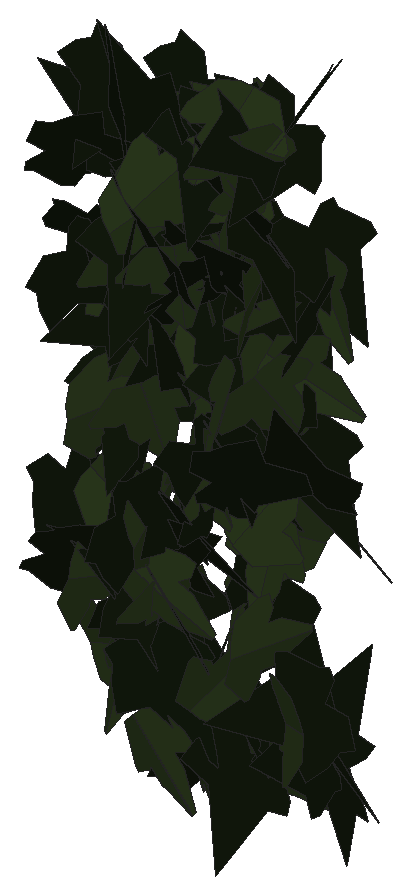
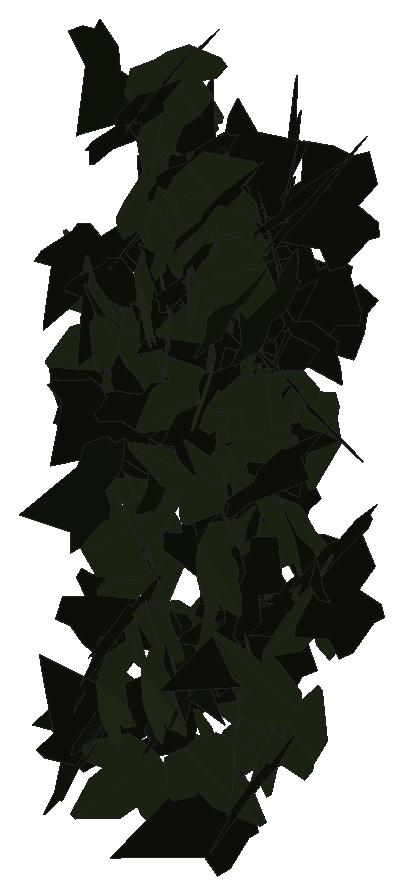
# SketchUp Ruby script. Lengths in inches.
U = 1.inch
M = Sketchup.active_model
def pt(a) = Geom::Point3d.new(a.map { |v| v * U })
def face(e, loops, mat)
  f = e.add_face(loops[0].map { |a| pt(a) })
  loops[1..].each { |l| e.add_face(l.map { |a| pt(a) }).erase! }
  f.material = f.back_material = mat if mat
  f
end
# faces: each face lists its corners as indices into pts; further lists are holes
def faces(e, pts, list, mat = nil) = list.each { |f| face(e, (f[0].is_a?(Array) ? f : [f]).map { |l| l.map { |i| pts[i] } }, mat) }
# xy, xz, yz: faces in a plane at the given z, y or x. An outline is a flat list of corners, or four numbers for a rectangle; further outlines are holes
def ring(l) = l.size == 4 ? [[l[0], l[1]], [l[2], l[1]], [l[2], l[3]], [l[0], l[3]]] : l.each_slice(2).to_a
def flat(e, list, mat, &to3) = list.each { |f| face(e, (f[0].is_a?(Array) ? f : [f]).map { |l| ring(l).map { |u, v| to3.(u, v) } }, mat) }
def xy(e, z, list, mat = nil) = flat(e, list, mat) { |x, y| [x, y, z] }
def xz(e, y, list, mat = nil) = flat(e, list, mat) { |x, z| [x, y, z] }
def yz(e, x, list, mat = nil) = flat(e, list, mat) { |y, z| [x, y, z] }
def lines(e, pts, list) = list.each { |a, b| e.add_line(pt(pts[a]), pt(pts[b])) }
# prism: a flat outline (further loops are holes) pulled along v
def prism(e, loops, v, mat = nil)
  f = face(e, loops, mat); d = Geom::Vector3d.new(v.map { |x| x * U })
  f.pushpull(f.normal.samedirection?(d) ? d.length : -d.length)
end
def box(e, o, s, mat = nil) = prism(e, [[o, [o[0] + s[0], o[1], o[2]], [o[0] + s[0], o[1] + s[1], o[2]], [o[0], o[1] + s[1], o[2]]]], [0, 0, s[2]], mat)
def at(x, y, z, deg = 0) = Geom::Transformation.translation(pt([x, y, z])) * Geom::Transformation.rotation(ORIGIN, Z_AXIS, deg.degrees)
def axes(o, x, y, z) = Geom::Transformation.new([*x, 0, *y, 0, *z, 0, *pt(o).to_a, 1])
def part(name) = M.definitions.add(name)
# library, detail: a bought-in or finely detailed component or shape, given as its bounding box
def library(name, o, s) = part(name).tap { |d| box(d.entities, o, s) }
def detail(e, o, s) = box(e.add_group.entities, o, s)
def put(e, d, t, mat = nil) = e.add_instance(d, t).tap { |i| i.material = mat if mat }
def group(e, t, mat = nil) = e.add_group.tap { |g| g.transformation = t; g.material = mat if mat }.entities
root = M.entities
M.materials.add("efeu1").color = [18, 25, 13]
M.materials.add("efeu2").color = [43, 57, 29]
c1 = part("ivyleaf_9")
p = [[1.54,2.16,1.25],[1.36,2.04,1.19],[-0.21,0.99,0.68],[-0.71,1.11,0.82],[-0.85,0.86,0.67],[-0.8,0.17,0.21],
  [-0.9,-0.01,0.1],[-0.67,-0.16,-0.02],[-0.08,-0.08,-0.05],[-0.03,-0.6,-0.4],[0.65,-0.88,-0.66],[0.83,-0.6,-0.49],
  [1.29,-0.42,-0.43],[1.8125,-0.07,-0.26],[1.21,0.44,0.15]]
faces(c1.entities,p,[[0,1,2,3,4,5,6,7,8,9,10,11,12,13,14]],"efeu1")
c2 = part("ivyleaf_10")
p = [[0,0.5,-0.03],[-0.0625,2.02,-0.43],[-0.19,2.01,-0.46],[-0.54,1.05,-0.29],[-0.52,0.625,-0.18],[-0.83,0.76,-0.28],
  [-1.16,0.64,-0.33],[-1.15,0.33,-0.24],[-0.77,-0.39,0.02],[-0.3,-0.51,0.16],[0.04,-0.48,0.23],[-0.02,2.01,-0.4375],
  [-0.06,2.01,-0.43],[0.04,-0.49,0.23],[0.67,-0.49,0.14],[1.38,0.36,-0.2],[1.375,0.51,-0.24],[0.81,0.65,-0.19],
  [0.62,0.59,-0.15],[0.6,1.09,-0.28],[0.5,1.23,-0.31]]
faces(c2.entities,p,[[0,1,2,3,4,5,6,7,8,9,10],[11,12,0,13,14,15,16,17,18,19,20]],"efeu2")
put(root,c1,axes([32.22,223.73,222.4],[-0.13186,-0.40837,0.25661],[-0.00992,-0.26368,-0.42471],[0.4822,-0.11709,0.06143]))
put(root,c1,axes([32.01,224.24,221.29],[0.17301,-0.3771,0.27904],[0.1407,-0.24201,-0.41429],[0.44752,0.22188,0.02237]))
put(root,c1,axes([32.44,223.46,221.91],[0.03944,-0.49844,-0.00094],[0.00497,-0.00055,0.49997],[-0.49842,-0.03945,0.00491]))
put(root,c1,axes([32.16,222.83,217.73],[0.19134,-0.43296,-0.16104],[-0.05637,0.15112,-0.47327],[0.45849,0.19927,0.00902]))
put(root,c1,axes([32.37,222.61,220.7],[0.03293,-0.1121,-0.48616],[-0.16207,0.45839,-0.11668],[0.47186,0.16527,-0.00615]))
put(root,c1,axes([32.77,223.26,219.95],[-0.43987,0.20202,0.12531],[-0.11789,0.04351,-0.48395],[-0.20644,-0.4553,0.00935]))
put(root,c2,axes([32.09,223.97,216.27],[0.27,-0.06732,-0.41541],[0.41343,-0.04972,0.27677],[-0.07858,-0.49295,0.02881]))
put(root,c1,axes([32.46,222.85,221.09],[0.39152,0.24878,-0.1866],[-0.16165,-0.09349,-0.46382],[-0.26567,0.42352,0.00723]))
put(root,c1,axes([32.17,222.54,221.96],[0.32807,0.12926,0.35449],[0.32971,0.13021,-0.35262],[-0.18347,0.46512,0.0002]))
put(root,c1,axes([32.43,223.93,218.93],[-0.12695,-0.43581,0.20964],[-0.05849,-0.20132,-0.45393],[0.48007,-0.13977,0.00013]))
put(root,c2,axes([32.19,223.37,215.35],[-0.2137,-0.01996,0.45159],[0.45203,-0.01193,0.21338],[0.00226,0.49946,0.02314]))
put(root,c1,axes([32.23,222.45,216.92],[0.38071,0.14901,0.28785],[0.27452,0.08787,-0.40856],[-0.17235,0.46912,-0.01491]))
put(root,c2,axes([32.51,223.63,219.96],[0.34227,0.36265,-0.0365],[-0.02577,-0.02586,-0.49867],[-0.36357,0.34324,0.00099]))
put(root,c1,axes([32.39,223.79,215.18],[0.25938,-0.37145,-0.21154],[-0.10155,0.18681,-0.45254],[0.41523,0.27772,0.02147]))
put(root,c2,axes([32.54,223.46,215.42],[0.00337,0.3534,-0.35369],[0.01589,-0.3536,-0.35315],[-0.49974,-0.00886,-0.01361]))
put(root,c2,axes([32.57,222.56,216.74],[-0.0455,-0.17923,-0.46455],[0.15204,0.4392,-0.18434],[0.47414,-0.15804,0.01453]))
put(root,c1,axes([32.45,223.27,220.65],[-0.22116,-0.1935,-0.40454],[0.34928,0.20856,-0.2907],[0.28124,-0.41117,0.04292]))
put(root,c1,axes([32.54,223.26,222.47],[0.00857,-0.06746,0.49535],[0.05202,-0.49262,-0.06799],[0.49721,0.05271,-0.00142]))
put(root,c1,axes([32.59,222.89,217.22],[-0.1893,0.25841,0.38392],[0.19952,-0.32869,0.31962],[0.41756,0.2742,0.02132]))
put(root,c2,axes([32.68,222.46,218.89],[-0.02048,-0.02386,-0.49901],[0.21752,0.44918,-0.0304],[0.44974,-0.21833,-0.00802]))
put(root,c1,axes([32.81,223.41,219.04],[-0.26869,-0.41923,-0.0453],[0.02902,0.0352,-0.49791],[0.42067,-0.27019,0.00542]))
put(root,c2,axes([33.22,223.69,219.16],[-0.05604,0.00247,-0.49684],[-0.49668,0.01284,0.05609],[0.01304,0.49983,0.00102]))
put(root,c1,axes([32.59,223.73,220.8],[-0.04495,-0.00015,0.49798],[0.27296,-0.4182,0.02451],[0.4165,0.27406,0.03768]))
put(root,c2,axes([32.87,223.1,220.68],[-0.30344,-0.36884,-0.14791],[0.09973,0.10946,-0.47757],[0.38468,-0.31933,0.00714]))
put(root,c1,axes([32.6,224.14,221.16],[0.1599,-0.42507,0.20915],[0.09948,-0.18569,-0.45346],[0.46318,0.18663,0.02519]))
put(root,c1,axes([33.1875,223.14,222.26],[0.05098,-0.06624,0.49296],[-0.32363,0.37189,0.08344],[-0.37771,-0.32758,-0.00495]))
put(root,c2,axes([32.79,223.49,216.18],[0.38359,-0.26646,0.17849],[0.1365,-0.11617,-0.46677],[0.29022,0.40682,-0.01637]))
put(root,c2,axes([32.62,223.89,221.5625],[-0.26985,-0.02007,-0.42045],[0.41366,-0.10504,-0.26048],[-0.07787,-0.48843,0.07329]))
put(root,c2,axes([33.1,223.41,215.26],[-0.04979,0.20582,-0.45295],[-0.16521,0.42254,0.21016],[0.46928,0.17059,0.02593]))
put(root,c2,axes([32.61,222.92,217.71],[0.27525,0.09269,0.407],[0.37494,0.15937,-0.28986],[-0.18346,0.46477,0.01823]))
put(root,c1,axes([32.82,223.26,221.78],[-0.22586,0.00093,-0.44608],[0.43434,-0.11348,-0.22015],[-0.10165,-0.48695,0.05046]))
put(root,c1,axes([32.92,224.31,222.32],[-0.0975,-0.41019,0.26878],[-0.01663,-0.27112,-0.41979],[0.49012,-0.09079,0.03923]))
put(root,c2,axes([33.19,224,215.07],[0.36889,0.11934,-0.31572],[-0.3114,-0.06009,-0.38655],[-0.13021,0.48182,0.02999]))
put(root,c2,axes([33.03,223.4,219.5],[-0.18576,-0.42583,-0.18482],[0.08653,0.16381,-0.46441],[0.45607,-0.20453,0.01284]))
put(root,c1,axes([32.86,223.07,216.38],[0.00673,0.1439,-0.4788],[0.04353,0.47685,0.14393],[0.49806,-0.04363,-0.00611]))
put(root,c2,axes([32.94,223.99,222.16],[0.48653,0.0864,0.07632],[0.07371,0.02133,-0.49408],[-0.08863,0.49202,0.00802]))
put(root,c1,axes([32.74,223.07,220.4375],[0.17681,0.00781,0.46763],[0.46702,0.02386,-0.17698],[-0.02508,0.49937,0.00115]))
put(root,c2,axes([33.08,223.96,217.69],[0.13905,-0.40963,0.25074],[0.09779,-0.23142,-0.4323],[0.47022,0.16926,0.01576]))
put(root,c1,axes([33.22,223.92,219.61],[-0.0157,-0.00422,-0.49974],[0.13726,-0.48079,-0.00025],[-0.48054,-0.13719,0.01626]))
put(root,c2,axes([33.21,222.91,219.07],[-0.30968,-0.3717,-0.12624],[0.08204,0.09596,-0.4838],[0.38388,-0.32036,0.00156]))
put(root,c2,axes([33.48,223.64,222.25],[-0.28751,-0.17244,0.37095],[-0.25986,-0.27317,-0.3284],[0.31592,-0.38163,0.06746]))
put(root,c1,axes([33.24,223.09,221.03],[-0.30496,-0.39501,-0.03108],[0.01923,0.02441,-0.49903],[0.39577,-0.30556,0.0003]))
put(root,c2,axes([33.06,222.75,221.33],[0.09851,0.14902,-0.467],[0.28931,0.36685,0.17809],[0.39572,-0.3053,-0.01395]))
put(root,c2,axes([33.35,222.61,217.53],[-0.01252,0.13295,-0.48184],[-0.00073,0.48198,0.13301],[0.49984,0.00403,-0.01187]))
put(root,c2,axes([33.17,223.6,221.27],[-0.44325,0.08071,-0.21683],[0.20736,-0.06927,-0.44967],[-0.10262,-0.48856,0.02793]))
put(root,c2,axes([33.04,223.44,220.8],[-0.18026,-0.11554,-0.45184],[0.40321,0.20482,-0.21324],[0.23436,-0.44125,0.01933]))
put(root,c2,axes([33.37,223.1875,216.55],[-0.12657,-0.48371,0.0007],[0.00137,-0.00108,-0.5],[0.48371,-0.12657,0.0016]))
put(root,c1,axes([33.3,222.33,217.8125],[0.08217,-0.00065,-0.4932],[-0.20009,0.45696,-0.03393],[0.45079,0.20294,0.07484]))
put(root,c1,axes([33.33,224.1,221.34],[-0.13886,-0.40408,0.2597],[-0.08649,-0.24488,-0.42726],[0.47248,-0.16358,-0.00189]))
put(root,c1,axes([33.23,223.21,216.52],[-0.12461,-0.41189,-0.2546],[0.07839,0.24227,-0.4303],[0.47784,-0.14716,0.0042]))
put(root,c1,axes([33.16,223.36,219.56],[0.02502,-0.24404,0.43568],[0.08855,-0.42715,-0.24435],[0.49146,0.08939,0.02184]))
put(root,c1,axes([33.01,223.25,216.99],[0.43726,0.02162,-0.24152],[0.23155,0.11064,0.42912],[0.07199,-0.48713,0.08674]))
put(root,c1,axes([33.5,222.91,220.7],[0.2532,-0.31882,0.29025],[-0.17894,0.22854,0.40712],[-0.39227,-0.31004,0.00164]))
put(root,c2,axes([33.29,223.8,220.03],[-0.25862,0.35922,-0.23254],[0.14363,-0.18308,-0.44255],[-0.4031,-0.2957,-0.00849]))
put(root,c1,axes([33.2,223.51,214.25],[0.30613,0.22764,0.32321],[0.26389,0.18672,-0.38144],[-0.29436,0.40413,-0.00583]))
put(root,c2,axes([33.54,223.68,221.59],[0.10599,-0.35871,-0.3318],[-0.09051,0.31923,-0.37403],[0.48018,0.13935,0.00274]))
put(root,c1,axes([33.2,223.62,220.31],[-0.13033,-0.03334,0.48156],[0.47226,-0.11205,0.12006],[0.09991,0.48614,0.0607]))
put(root,c2,axes([33.21,222.89,216.81],[-0.28053,-0.00857,-0.4138],[0.41198,-0.0537,-0.27819],[-0.03967,-0.49703,0.03719]))
put(root,c2,axes([33.32,222.82,214.88],[-0.35189,0.11017,-0.3377],[0.30332,-0.15417,-0.36637],[-0.18485,-0.4627,0.04167]))
put(root,c1,axes([33.94,223.37,221.9],[-0.22515,0.02017,-0.44598],[-0.2932,-0.38335,0.13068],[-0.33666,0.32037,0.18445]))
put(root,c2,axes([33.17,223.98,218.69],[0.05007,-0.07497,-0.4918],[0.49106,-0.07177,0.06094],[-0.07973,-0.48911,0.06644]))
put(root,c2,axes([33.92,223.83,221.7],[-0.17584,0.0686,0.46301],[-0.45624,0.08535,-0.18591],[-0.10454,-0.48786,0.03258]))
put(root,c1,axes([34,223.6,220.02],[-0.22325,0.06425,0.44275],[-0.42573,0.12157,-0.23231],[-0.13751,-0.48072,0.00043]))
put(root,c1,axes([33.35,222.87,215.91],[-0.13204,-0.15965,-0.45506],[0.34821,0.29485,-0.20448],[0.33364,-0.37091,0.03332]))
put(root,c2,axes([33.67,222.875,220.97],[-0.35368,-0.35018,-0.04781],[0.03312,0.0345,-0.49771],[0.35188,-0.35522,-0.0012]))
put(root,c1,axes([33.3,223.19,216.41],[0.17208,-0.29977,0.36129],[0.19126,-0.30664,-0.34553],[0.42873,0.25712,0.00913]))
put(root,c2,axes([33.44,222.67,221.83],[0.18458,0.19953,-0.41966],[0.28861,0.30468,0.2718],[0.36419,-0.34258,-0.0027]))
put(root,c1,axes([33.32,223.22,217.44],[0.34,-0.23541,0.28104],[0.2312,-0.15978,-0.41354],[0.28451,0.41116,0.0002]))
put(root,c2,axes([33.4,223.66,219.63],[0.27811,0.11116,0.40037],[0.33544,0.22426,-0.29527],[-0.24522,0.43284,0.05016]))
put(root,c1,axes([33.66,222.88,220.57],[0.23905,0.31581,0.30515],[0.17773,0.24813,-0.39603],[-0.40158,0.29781,0.00637]))
put(root,c2,axes([33.55,223.36,214.67],[-0.16298,0.15776,-0.44559],[0.28298,-0.34498,-0.22564],[-0.37863,-0.32573,0.02316]))
put(root,c1,axes([33.74,223.52,222.38],[-0.12419,-0.48116,0.05536],[-0.015,-0.05331,-0.49692],[0.4841,-0.12508,-0.00119]))
put(root,c1,axes([34.15,222.92,218.09],[-0.20324,0.30258,0.34226],[-0.18596,0.28736,-0.36448],[-0.41727,-0.27544,-0.00428]))
put(root,c2,axes([33.78,224.1,215.91],[0.17323,-0.3852,0.2676],[0.10453,-0.24639,-0.42233],[0.45724,0.20227,-0.00483]))
put(root,c2,axes([34.18,223.42,221.76],[0.18047,0.032,-0.4652],[-0.46569,-0.01296,-0.18155],[-0.02368,0.49881,0.02512]))
put(root,c2,axes([34.24,223.72,220.09],[0.09689,0.05738,-0.48715],[-0.4883,0.05847,-0.09023],[0.04661,0.49324,0.06737]))
put(root,c2,axes([33.73,223.95,220.63],[-0.13743,0.15364,-0.45553],[0.14912,-0.43678,-0.19231],[-0.45703,-0.18872,0.07423]))
put(root,c1,axes([33.91,223.55,216.12],[-0.29671,0.17721,-0.36133],[0.29965,-0.20239,-0.34532],[-0.26865,-0.42147,0.0139]))
put(root,c1,axes([33.93,223.52,221.39],[0.42508,0.07022,-0.25372],[-0.25105,-0.03693,-0.43082],[-0.07925,0.49366,0.00386]))
put(root,c1,axes([33.68,223.74,215.53],[0.23291,-0.4302,0.10333],[0.05687,-0.08669,-0.48913],[0.43877,0.2396,0.00855]))
put(root,c2,axes([34.05,223.7,216.39],[0.3627,-0.28777,-0.18877],[-0.1269,0.1431,-0.46197],[0.31991,0.38302,0.03077]))
put(root,c2,axes([33.93,224.1,220.96],[0.22985,-0.40771,0.17591],[0.12015,-0.13358,-0.4666],[0.42747,0.25677,0.03656]))
put(root,c2,axes([34.01,224.21,222.05],[-0.16423,0.1237,0.45577],[0.17078,-0.43433,0.17942],[0.4403,0.2146,0.10041]))
put(root,c2,axes([33.74,223.1,218.3125],[0.13636,-0.02145,0.48057],[0.46622,-0.11716,-0.13752],[0.11851,0.48561,-0.01195]))
put(root,c1,axes([33.76,223.07,220.92],[0.43942,0.03451,-0.23606],[0.23517,0.02051,0.44077],[0.0401,-0.49839,0.00179]))
put(root,c1,axes([34.09,223.25,221.63],[0.42997,-0.22189,0.12606],[-0.1082,0.06518,0.48378],[-0.23113,-0.4433,0.00803]))
put(root,c1,axes([33.87,223.03,218.58],[0.00563,-0.0363,-0.49865],[0.33108,0.37394,-0.02348],[0.37464,-0.32992,0.02824]))
put(root,c1,axes([34.19,223.78,219.32],[-0.31121,-0.38215,-0.08432],[0.05713,0.06222,-0.49281],[0.38715,-0.31637,0.00494]))
put(root,c1,axes([33.94,223.64,218.3],[0.077,-0.34204,0.35648],[0.13907,-0.33119,-0.34781],[0.47406,0.15271,0.04414]))
put(root,c2,axes([34.31,223.43,221.84],[0.03906,-0.45168,0.21085],[0.04782,-0.20713,-0.45256],[0.49617,0.05552,0.02702]))
put(root,c2,axes([34.2,222.79,215.66],[-0.08494,-0.34296,0.35378],[0.0827,0.34399,0.35332],[-0.48574,0.11854,-0.00171]))
put(root,c2,axes([34.33,222.89,219.56],[0.31807,-0.38577,0.00354],[0.00227,-0.00272,-0.49999],[0.38578,0.31807,0.00002]))
put(root,c1,axes([34.25,223.4,216.68],[-0.22544,0.36665,0.25445],[0.10778,-0.2319,0.42965],[0.43308,0.24857,0.02552]))
put(root,c2,axes([34.46,223.02,223.1],[0.35559,0.25894,-0.23771],[-0.20111,-0.12745,-0.43967],[-0.28829,0.4083,0.01351]))
put(root,c1,axes([34.78,223.55,219.58],[-0.09496,-0.04244,-0.48906],[-0.45284,-0.18473,0.10396],[-0.18951,0.46268,-0.00335]))
put(root,c2,axes([34.2,223.86,214.55],[-0.36382,-0.05584,-0.3384],[0.33433,0.05237,-0.36808],[0.07655,-0.49411,-0.00077]))
put(root,c1,axes([34.35,223.29,214.72],[-0.08994,-0.47586,0.12438],[-0.02105,-0.1226,-0.48428],[0.49139,-0.09235,0.00201]))
put(root,c2,axes([34.69,223.88,217.34],[-0.17809,-0.11127,-0.45377],[-0.34194,-0.29987,0.20773],[-0.31837,0.38431,0.03072]))
put(root,c2,axes([34.57,223.67,220.1875],[-0.1768,-0.41568,0.21436],[-0.05319,-0.2098,-0.45072],[0.46466,-0.18218,0.02997]))
put(root,c2,axes([34.7,222.8,220.83],[0.01678,-0.10441,-0.48869],[-0.11187,0.47577,-0.10549],[0.48704,0.11288,-0.00739]))
put(root,c2,axes([34.6,222.875,222.7],[-0.30715,-0.38191,-0.09902],[0.0642,0.07544,-0.49009],[0.38928,-0.31378,0.0027]))
put(root,c1,axes([34.34,223.52,221.44],[0.19873,-0.45787,0.02938],[0.01338,-0.02622,-0.49913],[0.45861,0.19917,0.00183]))
put(root,c1,axes([34.42,223.73,216.47],[0.25418,-0.36754,-0.2243],[-0.1121,0.195,-0.44655],[0.41573,0.27729,0.01673]))
put(root,c1,axes([34.59,223.21,222.71],[-0.17348,-0.19757,0.42529],[-0.0851,-0.43267,-0.23571],[0.46115,-0.15417,0.11649]))
put(root,c2,axes([34.52,223.98,215.5],[0.1438,-0.31478,0.36088],[0.16375,-0.32176,-0.34591],[0.45001,0.21768,0.01055]))
put(root,c1,axes([34.47,223.64,220.7],[-0.08389,-0.31408,-0.37989],[0.08004,0.37156,-0.32487],[0.48637,-0.11531,-0.01206]))
put(root,c1,axes([34.64,223.68,222.62],[-0.1464,-0.41928,0.22972],[-0.08412,-0.21391,-0.44404],[0.47063,-0.16867,-0.00791]))
put(root,c2,axes([34.7,223.25,217.68],[0.49071,-0.09583,-0.00455],[-0.00305,0.00812,-0.49992],[0.09589,0.49066,0.00738]))
put(root,c2,axes([34.57,223.02,217.82],[0.42041,-0.04119,-0.26751],[0.26928,0.01382,0.42106],[-0.02729,-0.49811,0.0338]))
put(root,c1,axes([35.09,223.5,220.48],[-0.36592,0.33767,-0.0456],[0.03367,-0.03075,-0.49792],[-0.33907,-0.36747,-0.00024]))
put(root,c1,axes([34.52,222.53,218.6],[0.29875,0.06843,0.39505],[0.38418,0.09206,-0.30648],[-0.11468,0.48666,0.00243]))
put(root,c1,axes([34.73,223.91,221.22],[-0.00761,-0.35301,-0.35402],[0.01514,0.35373,-0.35305],[0.49971,-0.0161,0.0053]))
put(root,c1,axes([35.01,223.23,222.98],[0.07888,0.31627,0.37914],[-0.00953,0.38485,-0.31906],[-0.49365,0.04311,0.06674]))
put(root,c2,axes([34.88,222.875,219.79],[-0.20844,-0.36478,-0.27108],[0.13697,0.23395,-0.42013],[0.43335,-0.2494,0.0024]))
put(root,c2,axes([34.85,222.59,216.56],[-0.03148,-0.0756,-0.49325],[0.17104,0.46266,-0.08183],[0.46878,-0.17388,-0.00327]))
put(root,c1,axes([34.79,223.77,214.69],[-0.18454,-0.14406,0.4418],[0.42175,0.14767,0.22432],[-0.19511,0.45546,0.06701]))
put(root,c1,axes([34.67,223.95,218.02],[0.39393,-0.26424,0.15808],[0.13009,-0.08984,-0.47435],[0.27909,0.41485,-0.00203]))
put(root,c2,axes([34.76,223.42,219.72],[0.19654,0.07536,0.45353],[0.37379,0.26098,-0.20535],[-0.26768,0.41977,0.04625]))
put(root,c1,axes([34.86,224.14,214.46],[0.13636,-0.4032,0.26237],[0.07636,-0.25111,-0.42557],[0.47495,0.15613,-0.00691]))
put(root,c1,axes([35.14,223.65,214.87],[-0.11683,-0.11316,0.47281],[-0.16253,-0.44919,-0.14767],[0.45819,-0.1882,0.06817]))
put(root,c2,axes([34.79,223.96,220.625],[0.28422,-0.04474,0.40892],[0.40397,-0.06345,-0.28772],[0.07763,0.49394,0.00008]))
put(root,c1,axes([34.81,223.72,215.24],[0.37016,-0.3162,0.11399],[0.08794,-0.07255,-0.48683],[0.32441,0.38046,0.00191]))
put(root,c2,axes([35.41,222.71,215.71],[0.12179,-0.0888,-0.47674],[-0.32934,0.34565,-0.14852],[0.35595,0.3502,0.0257]))
put(root,c1,axes([34.88,223.57,218.83],[-0.14572,-0.17601,-0.44473],[0.3497,0.27797,-0.22459],[0.32631,-0.3765,0.04209]))
put(root,c1,axes([35.54,223.06,215.91],[-0.07407,-0.08295,-0.48748],[-0.35186,-0.33749,0.11089],[-0.34743,0.35947,-0.00838]))
put(root,c1,axes([35.25,223.18,218.51],[0.43766,-0.10093,0.2197],[-0.21426,0.0486,0.44915],[-0.11202,-0.48729,-0.00071]))
